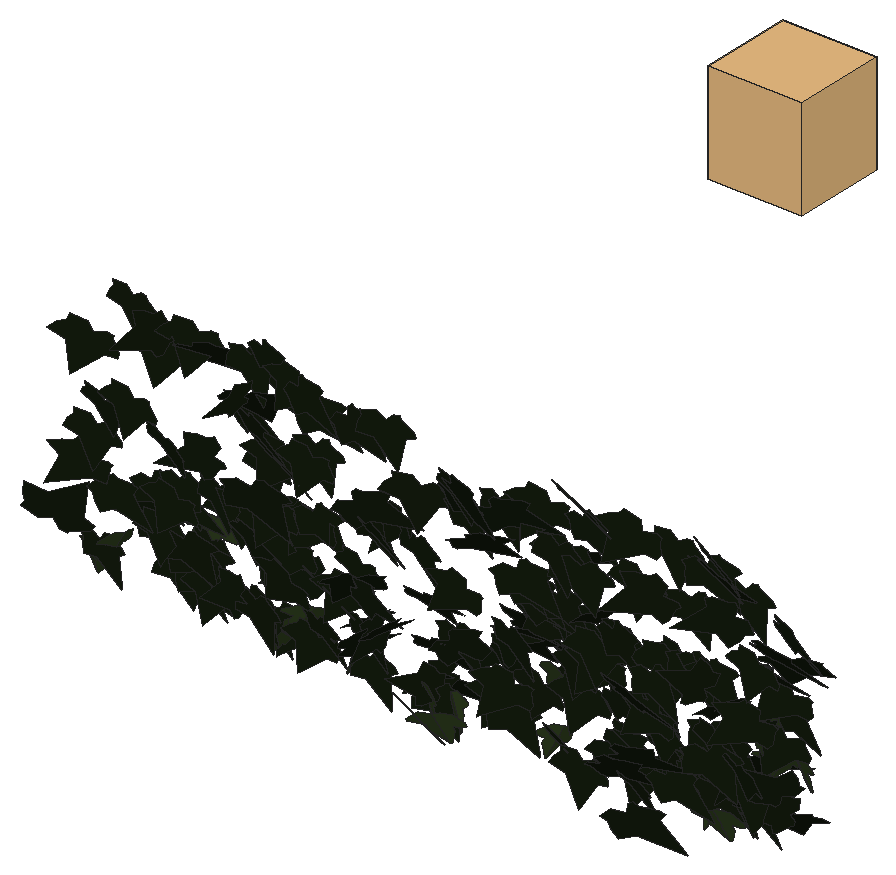
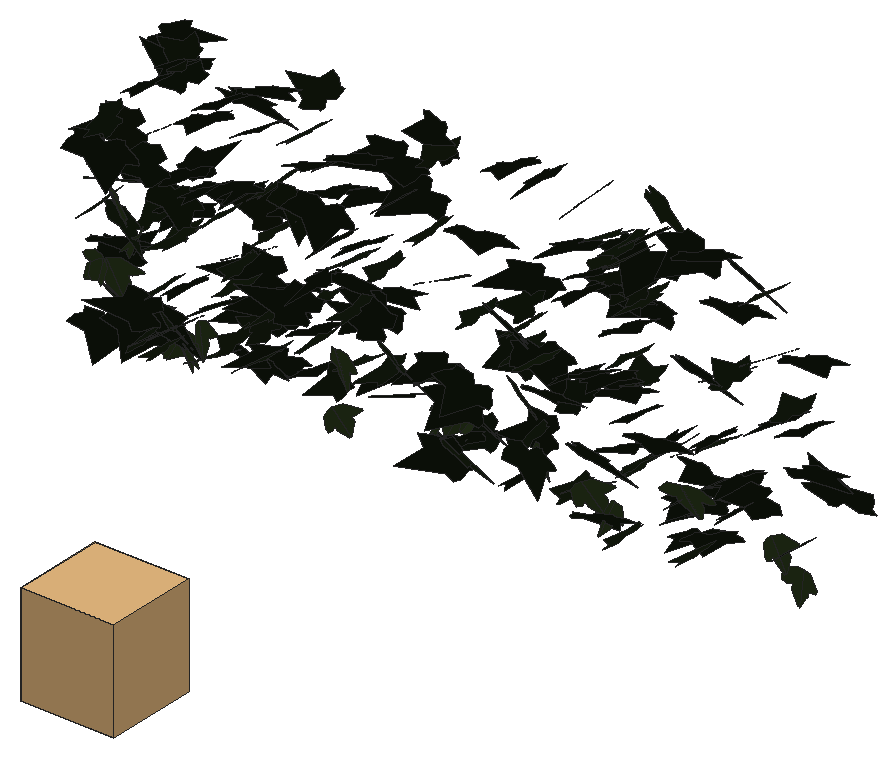
# SketchUp Ruby script. Lengths in millimetres.
U = 1.mm
M = Sketchup.active_model
def pt(a) = Geom::Point3d.new(a.map { |v| v * U })
def face(e, loops, mat)
  f = e.add_face(loops[0].map { |a| pt(a) })
  loops[1..].each { |l| e.add_face(l.map { |a| pt(a) }).erase! }
  f.material = f.back_material = mat if mat
  f
end
# faces: each face lists its corners as indices into pts; further lists are holes
def faces(e, pts, list, mat = nil) = list.each { |f| face(e, (f[0].is_a?(Array) ? f : [f]).map { |l| l.map { |i| pts[i] } }, mat) }
# xy, xz, yz: faces in a plane at the given z, y or x. An outline is a flat list of corners, or four numbers for a rectangle; further outlines are holes
def ring(l) = l.size == 4 ? [[l[0], l[1]], [l[2], l[1]], [l[2], l[3]], [l[0], l[3]]] : l.each_slice(2).to_a
def flat(e, list, mat, &to3) = list.each { |f| face(e, (f[0].is_a?(Array) ? f : [f]).map { |l| ring(l).map { |u, v| to3.(u, v) } }, mat) }
def xy(e, z, list, mat = nil) = flat(e, list, mat) { |x, y| [x, y, z] }
def xz(e, y, list, mat = nil) = flat(e, list, mat) { |x, z| [x, y, z] }
def yz(e, x, list, mat = nil) = flat(e, list, mat) { |y, z| [x, y, z] }
def lines(e, pts, list) = list.each { |a, b| e.add_line(pt(pts[a]), pt(pts[b])) }
# prism: a flat outline (further loops are holes) pulled along v
def prism(e, loops, v, mat = nil)
  f = face(e, loops, mat); d = Geom::Vector3d.new(v.map { |x| x * U })
  f.pushpull(f.normal.samedirection?(d) ? d.length : -d.length)
end
def box(e, o, s, mat = nil) = prism(e, [[o, [o[0] + s[0], o[1], o[2]], [o[0] + s[0], o[1] + s[1], o[2]], [o[0], o[1] + s[1], o[2]]]], [0, 0, s[2]], mat)
def at(x, y, z, deg = 0) = Geom::Transformation.translation(pt([x, y, z])) * Geom::Transformation.rotation(ORIGIN, Z_AXIS, deg.degrees)
def axes(o, x, y, z) = Geom::Transformation.new([*x, 0, *y, 0, *z, 0, *pt(o).to_a, 1])
def part(name) = M.definitions.add(name)
# library, detail: a bought-in or finely detailed component or shape, given as its bounding box
def library(name, o, s) = part(name).tap { |d| box(d.entities, o, s) }
def detail(e, o, s) = box(e.add_group.entities, o, s)
def put(e, d, t, mat = nil) = e.add_instance(d, t).tap { |i| i.material = mat if mat }
def group(e, t, mat = nil) = e.add_group.tap { |g| g.transformation = t; g.material = mat if mat }.entities
root = M.entities
M.materials.add("efeu1").color = [18, 25, 13]
M.materials.add("efeu2").color = [43, 57, 29]
c1 = part("ivyleaf_9")
p = [[39.1,54.8,31.7],[34.5,51.8,30.2],[-5.3,25.2,17.3],[-17.9,28.3,20.9],[-21.6,21.7,17],[-20.2,4.3,5.3],
  [-22.9,-0.3,2.5],[-17.1,-4,-0.6],[-2,-2.1,-1.2],[-0.7,-15.4,-10.1],[16.6,-22.3,-16.7],[21.1,-15.1,-12.5],
  [32.7,-10.7,-11],[46.1,-1.8,-6.6],[30.8,11.2,3.8]]
faces(c1.entities,p,[[0,1,2,3,4,5,6,7,8,9,10,11,12,13,14]],"efeu1")
c2 = part("ivyleaf_10")
p = [[0,12.8,-0.8],[-1.5,51.3,-10.9],[-4.9,51,-11.6],[-13.6,26.5,-7.3],[-13.2,15.9,-4.6],[-21.1,19.3,-7.2],
  [-29.5,16.3,-8.3],[-29.2,8.3,-6.2],[-19.7,-9.8,0.5],[-7.6,-13,4],[1,-12.2,5.8],[-0.4,51.1,-11.1],
  [-1.5,51.1,-10.9],[1,-12.4,5.9],[16.9,-12.4,3.5],[35.1,9.1,-5.1],[35,12.9,-6.1],[20.5,16.4,-4.9],
  [15.8,15,-3.8],[15.3,27.6,-7.1],[12.8,31.3,-7.8]]
faces(c2.entities,p,[[0,1,2,3,4,5,6,7,8,9,10],[11,12,0,13,14,15,16,17,18,19,20]],"efeu2")
c3 = library("Spot Light\#4",[-129.6,-129.6,-280.7],[259.2,259.2,280.7])
put(root,c1,axes([4198.2,621.9,4453],[-2.17521,-0.56393,0.28451],[-0.49117,-0.11993,-1.27446],[1.09721,-1.17168,-0.00648]))
put(root,c2,axes([4187.2,653,4207.9],[-1.96458,0.66362,0.3006],[-0.53689,0.11655,-1.22602],[-1.27837,-1.06879,0.05295]))
put(root,c1,axes([4182.6,644.8,4747.2],[-1.77094,-0.96735,-0.03453],[0.07015,0.01245,-1.34212],[1.8409,-0.93106,0.01792]))
put(root,c1,axes([4173.7,525.1,4344.4],[-1.68412,0.35327,1.1592],[1.86407,-0.63675,0.94171],[1.35815,1.31199,0.14491]))
put(root,c1,axes([4219.9,612.5,4546.3],[-0.69913,-1.27771,0.14771],[-0.04871,-0.14633,-1.32938],[2.44746,-0.3679,0.01574]))
put(root,c1,axes([4222.4,626.1,4254.8],[0.32814,-1.25535,-0.14444],[-0.04891,0.14227,-1.26712],[2.40445,0.17422,-0.00606]))
put(root,c1,axes([4221.1,638.4,4594.8],[-0.17399,-1.04647,0.79155],[0.40634,-0.79476,-1.02606],[2.46395,0.05717,0.22511]))
put(root,c2,axes([4255.4,654.6,4265.7],[-0.51962,-1.21507,0.10633],[-0.08084,-0.09942,-1.24521],[2.31995,-0.27561,-0.01957]))
put(root,c1,axes([4288.6,655.5,4871.3],[-0.21454,-1.27477,0.33346],[0.08333,-0.33811,-1.27777],[2.50639,-0.09788,0.07102]))
put(root,c1,axes([4293.9,651.4,4365.3],[0.7941,0.11418,-1.19805],[1.20217,1.05853,0.32087],[1.9496,-0.69922,0.29012]))
put(root,c1,axes([4324.5,678.6,4416.3],[0.2224,-1.03055,-0.76501],[-0.07622,0.76487,-1.03649],[2.4415,0.11775,0.03733]))
put(root,c1,axes([4341.9,586.1,4664.6],[-0.84168,-1.19771,0.44407],[-0.01634,-0.46713,-1.26846],[2.43106,-0.41781,0.14522]))
put(root,c1,axes([4339.5,666.6,4331.3],[0.44349,-1.20813,-0.37403],[-0.07039,0.37366,-1.22996],[2.40596,0.23363,0.03296]))
put(root,c1,axes([4343,505.4,4484],[0.73383,-1.04531,-0.7256],[0.10638,0.77136,-1.08154],[2.41942,0.28313,0.26763]))
put(root,c1,axes([4421.8,580.6,4863.1],[-2.42111,0.60102,-0.08894],[0.14414,-0.0479,-1.40691],[-1.14729,-1.27433,0.01093]))
put(root,c1,axes([4395.2,634,4803],[-1.87419,-0.84722,-0.36204],[0.67064,0.14329,-1.29379],[1.62017,-1.03937,0.11674]))
put(root,c1,axes([4402.9,619.3,4363.2],[-0.63281,-1.20454,0.19011],[-0.08931,-0.18427,-1.24958],[2.31914,-0.33577,0.00375]))
put(root,c1,axes([4414,678.9,4241.6],[-0.85109,-1.11859,-0.4356],[0.21682,0.4232,-1.2037],[2.27431,-0.45894,-0.04826]))
put(root,c1,axes([4429.1,644.8,4468.3],[0.16814,-1.26485,-0.32961],[-0.13151,0.32538,-1.26714],[2.48418,0.10283,-0.04477]))
put(root,c1,axes([4422.5,595.2,4590.1],[0.21836,-1.05693,0.82305],[0.54807,-0.78729,-1.05115],[2.48991,0.26599,0.1592]))
put(root,c1,axes([4428.6,707.5,4207.5],[0.7171,-1.19637,-0.10522],[0.02586,0.11451,-1.25341],[2.28557,0.37406,0.04719]))
put(root,c2,axes([4463.7,707.8,4347.6],[2.32206,0.04788,-0.28919],[-0.5535,0.04286,-1.21988],[-0.06979,1.25315,0.05277]))
put(root,c1,axes([4429.4,619.1,4443.4],[1.28685,-0.93162,-0.66201],[0.11275,0.79673,-1.0607],[2.17221,0.51055,0.44724]))
put(root,c1,axes([4447.2,678.8,4236.6],[0.09817,-1.01345,-0.78375],[0.23939,0.7846,-1.00627],[2.4265,-0.0364,0.13098]))
put(root,c1,axes([4468,653.2,4298.1],[-0.5128,-0.92664,-0.92044],[0.77281,0.83381,-0.9583],[2.36256,-0.47387,0.11368]))
put(root,c1,axes([4481.1,687.8,4315.1],[-0.22243,-1.20869,0.31111],[-0.13571,-0.3055,-1.21366],[2.37149,-0.13085,-0.04027]))
put(root,c1,axes([4465.7,612.9,4346],[-0.80442,-0.47061,-1.11979],[2.02948,0.42397,-0.58068],[1.10696,-1.1193,0.25087]))
put(root,c1,axes([4547.4,601.6,4588.6],[-2.29914,0.44614,0.26944],[-0.49616,0.0717,-1.28759],[-0.85892,-1.23564,0.02257]))
put(root,c1,axes([4506,606,4876.9],[-1.42236,-1.12046,-0.07532],[0.06806,0.06669,-1.34682],[2.13619,-0.74817,-0.00724]))
put(root,c1,axes([4491.3,701,4446.1],[0.0135,-1.25666,0.16762],[-0.06924,-0.16776,-1.25614],[2.41187,0.00222,-0.037]))
put(root,c1,axes([4521.3,646.8,4236.8],[-0.82066,-1.17383,0.45924],[-0.17031,-0.45564,-1.24864],[2.39287,-0.43501,0.06863]))
put(root,c1,axes([4530.3,502.8,4518.2],[-1.11825,-1.04687,0.60097],[-0.11015,-0.64318,-1.17699],[2.29472,-0.54103,0.23637]))
put(root,c1,axes([4525.5,574.4,4862.4],[2.25203,0.61737,0.26006],[0.44223,0.11684,-1.33465],[-1.19581,1.20588,-0.00382]))
put(root,c1,axes([4559.2,694.6,4435.6],[-1.56947,-0.82912,-0.47806],[0.9349,0.17492,-1.15071],[1.56327,-0.93701,0.20821]))
put(root,c1,axes([4621.2,609.4,4738.4],[1.52482,-0.87049,-0.63857],[-0.3957,0.65591,-1.15498],[2.01622,0.78706,0.25626]))
put(root,c1,axes([4627.6,711.6,4180],[0.47682,-1.21851,0.13044],[0.03168,-0.12975,-1.24396],[2.33211,0.2509,-0.00977]))
put(root,c1,axes([4666.8,546.1,4310.7],[-0.71611,-0.3566,1.25662],[-1.27586,-1.06965,-0.50427],[2.13367,-0.75929,0.12022]))
put(root,c1,axes([4652,643.4,4446.1],[-0.25147,-1.30218,0.02339],[-0.01076,-0.02293,-1.30886],[2.47869,-0.13221,-0.00331]))
put(root,c1,axes([4671,686.7,4374.2],[-1.28492,-1.0514,0.26656],[-0.07988,-0.28842,-1.24393],[2.06278,-0.66609,0.11787]))
put(root,c1,axes([4653,607.9,4869.3],[-0.0984,-1.35294,-0.0195],[0.00207,0.01948,-1.35393],[2.57519,-0.05171,0.00034]))
put(root,c1,axes([4647.6,655.3,4846.4],[0.62704,-1.24322,-0.31249],[0.01769,0.32496,-1.28301],[2.43964,0.31718,0.08962]))
put(root,c1,axes([4657.1,660.4,4587.8],[-0.14463,-1.23712,0.38307],[0.10814,-0.38655,-1.23707],[2.46241,-0.05569,0.07683]))
put(root,c1,axes([4680.9,666.1,4503.6],[-1.39953,-1.04333,0.06805],[-0.0321,-0.07135,-1.27614],[1.98962,-0.73504,0.02728]))
put(root,c3,at(4681.1,2446,4806.3))
put(root,c1,axes([4655.1,649.7,4871.7],[1.0809,-1.17667,-0.19996],[-0.08032,0.20151,-1.30565],[2.27013,0.56739,0.04901]))
put(root,c1,axes([4679.1,565.6,4799.8],[2.15943,0.88787,-0.20203],[-0.31028,-0.11948,-1.44072],[-1.70499,1.14627,0.00631]))
put(root,c1,axes([4665.2,591.3,4295.3],[0.72383,-1.35861,-0.05097],[-0.0282,0.04878,-1.41084],[2.58737,0.38061,-0.00112]))
put(root,c1,axes([4668.8,587.6,4727],[1.22943,-1.18876,0.24908],[0.19959,-0.22647,-1.35284],[2.30294,0.65425,-0.01572]))
put(root,c1,axes([4686.5,583,4284.4],[0.30938,-1.39094,0.187],[-0.01497,-0.18915,-1.40009],[2.671,0.16005,-0.02951]))
put(root,c1,axes([4720.8,702.8,4194.2],[-1.8468,-0.78716,0.04801],[0.12187,-0.15452,-1.23918],[1.49596,-0.95919,0.16022]))
put(root,c2,axes([4710.2,647.7,4188.9],[-0.14665,-0.87526,-0.91098],[0.53193,0.87825,-0.86745],[2.34477,-0.25398,0.13981]))
put(root,c1,axes([4745.7,460.8,4867.2],[-1.6426,1.00778,-0.3785],[0.42183,-0.30838,-1.32648],[-2.00493,-0.89054,0.03101]))
put(root,c1,axes([4770.7,684.2,4332.9],[-2.24847,0.30894,0.32486],[-0.59642,0.08569,-1.22114],[-0.61014,-1.22227,-0.0035]))
put(root,c1,axes([4717.6,551.2,4461.4],[-0.73834,-0.87853,0.97421],[0.43475,-1.04564,-0.85198],[2.45853,-0.07893,0.44323]))
put(root,c2,axes([4755.3,683.8,4239.7],[-0.97077,-1.02092,0.52289],[-0.27127,-0.51141,-1.13754],[2.16612,-0.52158,0.09188]))
put(root,c1,axes([4772.8,575.9,4684.8],[-2.29057,-0.51015,-0.24264],[0.4059,0.11847,-1.30694],[0.99558,-1.22202,-0.02541]))
put(root,c1,axes([4743.1,613.9,4495.7],[-0.11946,-1.19796,-0.55241],[0.20864,0.54639,-1.19735],[2.502,-0.10276,0.07347]))
put(root,c1,axes([4768.1,633,4834.1],[-1.31021,-0.9011,0.6956],[-0.16576,-0.76883,-1.08217],[2.16016,-0.60555,0.33886]))
put(root,c1,axes([4776.1,538,4569.9],[-1.11249,-1.1918,0.42443],[-0.31188,-0.39228,-1.32721],[2.3875,-0.60658,0.0244]))
put(root,c1,axes([4735.3,558.3,4695.8],[1.44969,-1.13179,0.51572],[0.53232,-0.43338,-1.36421],[2.30648,0.81139,-0.00929]))
put(root,c1,axes([4788.9,576,4457.8],[-1.89015,-0.87565,-0.0172],[0.02347,0.01202,-1.32404],[1.66669,-0.99322,-0.00086]))
put(root,c1,axes([4749.4,491.3,4627.1],[-1.08951,-0.39235,-1.2628],[1.95688,0.7332,-0.69392],[1.58251,-1.17677,-0.01132]))
put(root,c1,axes([4797.7,647.4,4494.5],[-1.39903,-0.97402,0.41867],[-0.2092,-0.4367,-1.20895],[2.00687,-0.72453,0.16584]))
put(root,c1,axes([4803.3,648.9,4207.7],[-1.08796,-1.06868,0.43413],[-0.23206,-0.42582,-1.20878],[2.18304,-0.57786,0.08786]))
put(root,c1,axes([4784.6,679.9,4226.2],[0.78188,-1.15155,0.26388],[0.18512,-0.24546,-1.22261],[2.24081,0.42209,0.00893]))
put(root,c1,axes([4791.8,654.5,4509.4],[0.42885,-1.16194,-0.53232],[0.15788,0.55268,-1.17128],[2.4273,0.16934,0.17023]))
put(root,c1,axes([4812.1,635.7,4690.8],[-0.11072,-1.31597,-0.24903],[-0.03056,0.24993,-1.31699],[2.54882,-0.05417,-0.02661]))
put(root,c1,axes([4843.3,577.1,4698.3],[-0.99812,-1.14335,0.3608],[-0.11115,-0.36897,-1.25416],[2.27909,-0.51872,0.09684]))
put(root,c1,axes([4822.1,617,4798.9],[0.51809,-0.95711,-0.88866],[0.41506,0.92832,-0.93302],[2.45078,0.04511,0.34588]))
put(root,c1,axes([4840.9,544.5,4884.4],[1.02518,-1.10963,-0.68],[-0.44576,0.64127,-1.23197],[2.43641,0.58423,0.06073]))
put(root,c1,axes([4848.3,593.7,4387.5],[0.72853,-0.93172,0.93945],[0.90495,-0.81577,-1.00281],[2.34995,0.603,0.09492]))
put(root,c1,axes([4911.7,688,4277.2],[0.28555,1.27275,-0.06793],[-0.01066,-0.06774,-1.28156],[-2.42572,0.15012,-0.00236]))
put(root,c1,axes([4929.5,615.3,4389.5],[-2.17985,-0.51639,-0.17128],[0.48712,-0.15916,-1.23167],[0.91371,-1.14711,0.248]))
put(root,c2,axes([4932.6,629.1,4237],[0.82258,-1.13409,0.29773],[0.20642,-0.27729,-1.21366],[2.22197,0.4456,0.00252]))
put(root,c1,axes([4978.6,563.5,4452.7],[0.57934,1.14447,-0.73418],[-0.36633,-0.7085,-1.18425],[-2.56174,0.36014,0.00332]))
put(root,c1,axes([4935.9,648,4284.3],[0.61149,-1.2243,0.35256],[0.15775,-0.34274,-1.26574],[2.41963,0.33175,-0.00658]))
put(root,c1,axes([4945.8,656.7,4198.8],[0.20015,-1.30888,-0.29519],[-0.08566,0.29249,-1.31293],[2.5522,0.11246,-0.02092]))
put(root,c1,axes([4951.6,618.2,4453.6],[-0.41986,-1.11031,0.60959],[0.16828,-0.63076,-1.11686],[2.4048,-0.14971,0.18459]))
put(root,c1,axes([4944.9,580.2,4263],[0.79218,0.36053,1.25445],[1.74761,0.85487,-0.55037],[-1.76542,1.00802,0.01808]))
put(root,c1,axes([4949.8,640.8,4564.1],[0.7669,-1.21226,-0.24904],[-0.09611,0.24558,-1.27715],[2.35339,0.40507,0.029]))
put(root,c1,axes([4991.2,318.3,4555.7],[-1.38603,-0.69552,1.1133],[-0.06726,-1.2623,-0.81172],[2.49743,-0.42,0.596]))
put(root,c1,axes([5014.4,667.3,4569.5],[-2.17905,0.21205,-0.56374],[1.00198,-0.23585,-1.15795],[-0.55682,-1.25422,0.12243]))
put(root,c1,axes([4990.5,524.5,4873.4],[0.78902,-0.9867,-0.84246],[-0.3899,0.82354,-1.06536],[2.43829,0.45099,0.10225]))
put(root,c1,axes([4976,599.6,4580.5],[1.35017,-1.03812,0.32015],[0.32257,-0.27192,-1.2573],[2.04226,0.72927,-0.01307]))
put(root,c1,axes([4976.2,569.3,4640.5],[0.39665,-0.07674,-1.38118],[0.83252,1.32875,-0.00782],[2.49762,-0.43072,0.22195]))
put(root,c1,axes([5035.6,575.1,4339.2],[-1.94864,0.55738,-0.66076],[1.07879,-0.34044,-1.16551],[-1.24216,-1.17005,0.02435]))
put(root,c1,axes([5010.8,536.6,4446.7],[1.69584,-0.72957,-0.67448],[-0.58515,0.65904,-1.11906],[1.79816,0.90252,0.27194]))
put(root,c1,axes([5069.9,552.6,4880.6],[-0.44423,-1.27695,-0.30092],[0.10736,0.2956,-1.2981],[2.49455,-0.24012,0.00228]))
put(root,c1,axes([5069.8,686,4389.1],[2.33781,0.21743,-0.26564],[-0.52851,0.04919,-1.24385],[-0.38406,1.25579,0.09472]))
put(root,c1,axes([5076.1,501.1,4379.1],[1.08034,0.58795,1.0697],[1.07251,0.92024,-0.80484],[-2.06073,0.78717,0.14191]))
put(root,c1,axes([5078.4,652.6,4543],[0.37237,-1.25727,0.37387],[0.17066,-0.3643,-1.27201],[2.49054,0.21294,0.03127]))
put(root,c1,axes([5136.7,687.3,4218.7],[-2.02226,0.63676,-0.30987],[0.29098,-0.33928,-1.22149],[-1.31598,-1.05353,0.20608]))
put(root,c1,axes([5122.7,605.6,4712.3],[-1.69836,-0.80246,-0.52832],[0.7927,0.32666,-1.19967],[1.64777,-0.98425,0.03258]))
put(root,c1,axes([5180.5,577.7,4246.4],[-1.53447,0.80915,0.54487],[-0.71444,0.3951,-1.14221],[-1.71361,-0.88929,-0.0117]))
put(root,c1,axes([5125.3,647.5,4309.9],[2.31188,0.3756,-0.03514],[-0.06365,-0.01078,-1.27148],[-0.71513,1.21519,-0.00042]))
put(root,c1,axes([5123.9,551.2,4197.3],[2.08378,-0.57027,-0.27413],[-0.43558,0.15384,-1.23413],[1.12268,1.11815,0.02998]))
put(root,c1,axes([5117,689.3,4193.6],[2.21814,0.13479,0.4986],[0.93696,0.08229,-1.17302],[-0.2973,1.26498,0.02318]))
put(root,c2,axes([5159,584.2,4229.1],[-0.96697,1.01692,-0.54611],[0.34395,-0.51923,-1.13501],[-2.16974,-0.53551,0.06346]))
put(root,c1,axes([5152.6,627.8,4204.3],[-0.18253,-1.18698,-0.55787],[0.06122,0.55706,-1.19079],[2.49538,-0.10049,-0.01159]))
put(root,c1,axes([5187.2,652.5,4359],[0.41302,-1.24933,-0.14827],[0.1255,0.16155,-1.2647],[2.39113,0.20732,0.09199]))
put(root,c2,axes([5224.1,534.5,4206.1],[-2.1198,-0.5065,-0.34144],[0.57278,0.16288,-1.22335],[1.01165,-1.15353,-0.02281]))
put(root,c2,axes([5220.8,605.6,4217.6],[-0.3192,1.21082,-0.34158],[0.07086,-0.33967,-1.22234],[-2.39332,-0.17155,0.00937]))
put(root,c1,axes([5208,609.8,4359.4],[0.2025,-0.07283,-1.33171],[0.04762,1.33581,-0.07105],[2.53784,-0.01925,0.10759]))
put(root,c1,axes([5224.8,622.2,4692.6],[0.90889,-1.25207,-0.18062],[-0.10173,0.17292,-1.34],[2.40546,0.4804,0.01158]))
put(root,c1,axes([5270.3,572.9,4525.4],[-1.57561,-0.73034,0.72215],[-0.39876,-0.78794,-1.03707],[1.91363,-0.76552,0.37848]))
put(root,c1,axes([5335.1,657.5,4370.5],[-2.00904,0.65223,-0.3732],[0.55281,-0.23936,-1.23989],[-1.319,-1.09375,0.04879]))
put(root,c1,axes([5294,525.9,4802.4],[-0.10903,-1.07996,0.85608],[0.48775,-0.85023,-1.05542],[2.57708,0.11523,0.23597]))
put(root,c1,axes([5328.9,641.7,4252.4],[-1.50218,-0.92994,0.32794],[0.05774,-0.44276,-1.18252],[1.87581,-0.73109,0.29902]))
put(root,c1,axes([5299.2,671.9,4342.7],[1.50986,-1.01362,-0.28741],[-0.14541,0.30348,-1.2812],[1.9999,0.78732,0.12383]))
put(root,c1,axes([5322.9,635,4735.9],[0.23008,-1.33246,-0.04934],[-0.03737,0.04776,-1.33785],[2.53741,0.12152,-0.01523]))
put(root,c1,axes([5311.9,484.4,4832.3],[-0.02648,0.03691,-1.4553],[2.77057,0.0082,-0.01371],[0.01494,-1.45534,-0.03698]))
put(root,c1,axes([5335.1,510,4698.8],[2.12394,0.7508,0.52686],[0.83504,0.29168,-1.34504],[-1.53297,1.19913,-0.0027]))
put(root,c1,axes([5342.3,667.8,4429.4],[1.19644,-0.57449,0.99092],[1.39674,-0.66583,-0.8516],[1.67369,0.96633,0.00232]))
put(root,c1,axes([5380.3,607.3,4441.5],[2.48039,0.37645,0.03702],[0.06761,0.0104,-1.35655],[-0.71673,1.30376,0.00013]))
put(root,c1,axes([5383.3,590.7,4258.8],[-0.00447,-1.10531,-0.68086],[0.23731,0.67752,-1.10032],[2.45927,-0.06739,0.10494]))
put(root,c1,axes([5392.7,676.1,4460.9],[1.08954,-1.16183,-0.0931],[-0.0884,0.08091,-1.2952],[2.21653,0.57433,-0.00589]))
put(root,c1,axes([5384,537,4781.3],[0.13141,0.21885,-1.43136],[1.04973,1.32098,0.22858],[2.54806,-0.55549,-0.02035]))
put(root,c1,axes([5419.2,657.7,4303.2],[-0.80671,-1.07127,0.62758],[0.01297,-0.66514,-1.13079],[2.36291,-0.36209,0.22047]))
put(root,c2,axes([5442.8,679.6,4323.1],[1.59666,-0.77947,-0.52171],[-0.30155,0.57212,-1.10957],[1.75945,0.8054,0.28327]))
put(root,c2,axes([5445.2,686.2,4184.2],[-0.72322,-1.07178,0.54613],[0.095,-0.58629,-1.11586],[2.28739,-0.31452,0.21902]))
put(root,c1,axes([5423.8,601.1,4584.4],[0.52857,-1.12082,-0.60678],[0.17231,0.6368,-1.13483],[2.41955,0.1995,0.21337]))
put(root,c1,axes([5422.8,540.9,4486.6],[0.61918,-1.26749,0.32696],[0.15657,-0.31645,-1.30857],[2.48632,0.33557,0.00098]))
put(root,c1,axes([5476.5,641.5,4495.6],[-2.39039,-0.35142,0.02931],[-0.04722,-0.02008,-1.30416],[0.66948,-1.25617,0.01265]))
put(root,c1,axes([5469.2,491.8,4394.6],[-1.81564,-0.84654,0.23753],[-0.37912,-0.13328,-1.27503],[1.62985,-0.97404,-0.03197]))
put(root,c1,axes([5466.1,620.2,4787.8],[-1.72896,-0.9713,0.2073],[-0.10735,-0.23003,-1.32498],[1.88716,-0.90296,0.11455]))
put(root,c1,axes([5434.1,607.5,4546.7],[1.35452,-0.8815,-0.68058],[-0.09566,0.78144,-1.0647],[2.11735,0.59922,0.38728]))
put(root,c1,axes([5460,524.4,4658.7],[0.10465,-0.99872,-0.93345],[0.54873,0.92166,-0.96912],[2.5432,-0.15776,0.24751]))
put(root,c1,axes([5508.7,653,4660],[1.52284,1.02322,-0.25314],[-0.33885,-0.18204,-1.29863],[-1.97727,0.81925,0.02759]))
put(root,c1,axes([5481.7,613.7,4224.8],[1.92255,-0.77261,-0.12133],[-0.17612,0.07872,-1.27174],[1.478,1.01438,0.00628]))
put(root,c1,axes([5499.3,656.3,4499],[0.82296,-0.61036,-1.13884],[-0.66435,1.10108,-0.72267],[2.36767,0.52111,0.19306]))
put(root,c1,axes([5517.2,627.3,4689.8],[-1.09346,-1.19737,0.16548],[-0.03701,-0.17404,-1.32684],[2.3002,-0.572,0.05732]))
put(root,c1,axes([5512.4,687,4333.5],[-0.44076,-1.06441,0.75246],[-0.17497,-0.749,-1.08781],[2.47468,-0.24254,0.0571]))
put(root,c1,axes([5501,612.6,4571.3],[0.63576,-1.10321,-0.59625],[-0.19498,0.59097,-1.15084],[2.37868,0.3433,0.06503]))
put(root,c1,axes([5539.3,633.4,4401],[-0.40739,-1.01009,0.80251],[-0.10368,-0.80568,-1.02861],[2.45309,-0.2018,0.0898]))
put(root,c1,axes([5553.2,641.4,4338.5],[-1.12916,-1.21783,0.29633],[-0.17014,-0.28591,-1.35396],[2.37934,-0.59839,0.04381]))
put(root,c1,axes([5540.8,563.9,4728],[-0.15956,-1.38207,0.15317],[-0.01236,-0.15306,-1.38461],[2.64643,-0.08404,0.00277]))
put(root,c1,axes([5547.2,679.4,4401.8],[0.70023,-0.11223,1.30728],[2.45593,0.27669,-0.33942],[-0.45198,1.32959,0.18098]))
put(root,c1,axes([5602.9,647,4426.7],[-1.55866,-0.913,0.44209],[-0.26077,-0.46342,-1.21086],[1.91291,-0.80709,0.19515]))
put(root,c1,axes([5590.7,583.2,4202.3],[-0.64786,-1.32051,0.19637],[-0.10454,-0.18863,-1.36367],[2.53869,-0.34475,-0.00604]))
put(root,c1,axes([5587.8,595.9,4798.5],[0.77309,-1.22151,-0.33495],[0.02926,0.35648,-1.28139],[2.41041,0.38745,0.12298]))
put(root,c1,axes([5602,563.7,4698.5],[-0.68415,-1.24355,-0.26908],[0.62085,0.18018,-1.26853],[2.34055,-0.41129,0.25784]))
put(root,c1,axes([5583.4,556.9,4865.8],[0.68678,-0.99137,0.89218],[0.98827,-0.7469,-1.03996],[2.33804,0.60692,0.17751]))
put(root,c1,axes([5640.5,568.6,4597.3],[0.70644,1.26574,0.06994],[0.04834,0.06543,-1.31903],[-2.41215,0.372,-0.00595]))
put(root,c1,axes([5633.4,635.8,4366.1],[1.41068,-0.91425,-0.59007],[-0.47229,0.55312,-1.16873],[2.01637,0.76918,0.13907]))
put(root,c1,axes([5635,651.1,4261.3],[1.39552,-0.84139,-0.73851],[-0.33566,0.78497,-1.06944],[2.10407,0.68328,0.31921]))
put(root,c1,axes([5631.2,636.9,4241.6],[0.4056,-0.46274,-1.28453],[0.85987,1.25074,-0.37561],[2.45211,-0.36205,0.34418]))
put(root,c1,axes([5674.7,541.5,4547.3],[-1.15592,-1.15631,-0.13362],[0.12895,0.11534,-1.3061],[2.21158,-0.61109,0.00632]))
put(root,c1,axes([5662.6,626.5,4532.5],[0.28917,-1.31759,0.25893],[0.07528,-0.25607,-1.32629],[2.55449,0.1567,0.00978]))
put(root,c1,axes([5718.7,636.9,4212],[-2.08416,-0.1847,-0.62254],[1.15704,0.13734,-1.11015],[0.43433,-1.25216,-0.02993]))
put(root,c1,axes([5752.8,578.6,4834.7],[-1.90703,-0.86953,0.39492],[-0.39061,-0.36297,-1.31993],[1.77511,-1.01402,0.13382]))
put(root,c1,axes([5722.9,530.2,4596.3],[1.02527,-1.31162,-0.38333],[-0.24464,0.36157,-1.41783],[2.58917,0.55355,0.01783]))
put(root,c1,axes([5725.2,687.9,4261.7],[0.4412,-1.144,0.52617],[0.16822,-0.51891,-1.16716],[2.39061,0.24765,-0.01498]))
put(root,c1,axes([5718.3,500.3,4280.1],[2.25026,0.20201,0.70448],[1.32151,0.11895,-1.19949],[-0.44616,1.37117,0.00027]))
put(root,c1,axes([5734.2,559.3,4235.3],[0.85988,-1.18045,0.63929],[0.52632,-0.57821,-1.26312],[2.50014,0.52772,0.04604]))
put(root,c1,axes([5764.4,571.6,4729.3],[-0.70054,-1.28406,0.32494],[-0.04119,-0.33138,-1.33402],[2.52052,-0.3623,0.06851]))
put(root,c1,axes([5749,632.6,4420.6],[0.74701,-1.23269,0.17099],[0.08037,-0.166,-1.29363],[2.36716,0.39464,-0.01004]))
put(root,c1,axes([5803.4,575.5,4403.8],[-1.45221,-0.75243,0.82337],[-0.5608,-0.82617,-1.02807],[2.04738,-0.76,0.30241]))
put(root,c1,axes([5789.4,706.3,4210.3],[-0.92016,-1.06031,0.46299],[0.09244,-0.51994,-1.14002],[2.20002,-0.42163,0.24154]))
put(root,c1,axes([5784.9,615.1,4343.8],[-0.38608,-1.13699,0.59075],[0.17626,-0.60956,-1.14138],[2.4322,-0.13631,0.17649]))
put(root,c2,axes([5806.5,703.3,4275.5],[-0.00615,-1.20526,-0.37549],[0.10058,0.37503,-1.20425],[2.40049,-0.0188,0.0495]))
put(root,c1,axes([5765.2,493.1,4483.2],[1.41917,-0.8168,0.88263],[1.30023,-0.56696,-1.10184],[1.88356,1.00679,0.09558]))
put(root,c1,axes([5814.4,644.8,4519.8],[-0.35753,-1.15985,0.59786],[-0.14041,-0.59361,-1.1748],[2.47945,-0.20086,0.01968]))
put(root,c1,axes([5815.9,630.6,4806.7],[-0.55943,-1.31968,0.07818],[0.00058,-0.08016,-1.3519],[2.51601,-0.29341,0.0177]))
put(root,c1,axes([5777.9,493,4327.5],[1.92282,0.04668,0.96525],[1.82655,0.11508,-1.0101],[-0.2154,1.39255,0.05112]))
put(root,c1,axes([5870.1,503,4749.9],[-2.59938,-0.0259,0.33043],[-0.62875,-0.00669,-1.36604],[0.0509,-1.40518,0.00041]))
put(root,c1,axes([5832.5,520.9,4534.1],[0.21257,-1.19892,-0.53814],[-0.0873,0.53619,-1.20411],[2.49958,0.12068,0.00371]))
put(root,c1,axes([5818.1,460.6,4207.6],[-0.01193,-0.34959,-1.30411],[1.35913,1.10591,-0.29989],[2.18074,-0.69116,0.17977]))
put(root,c1,axes([5848.6,572.7,4560.6],[-1.32008,-1.22984,-0.3321],[0.31451,0.28807,-1.41194],[2.40397,-0.71302,0.00236]))
put(root,c1,axes([5847.4,560.4,4267.8],[0.8395,-1.0599,-0.73058],[0.16415,0.79488,-1.10111],[2.44449,0.31062,0.32484]))
put(root,c1,axes([5875.5,667.2,4347.9],[0.12194,-1.26811,-0.30251],[-0.09526,0.30026,-1.26928],[2.47936,0.0739,-0.03389]))
put(root,c2,axes([5893.3,655.2,4179.2],[1.51392,-0.92167,0.22736],[0.27072,-0.17755,-1.21744],[1.7863,0.80804,-0.00818]))
put(root,c1,axes([5878.4,594.2,4552.5],[0.13549,-1.25881,-0.39591],[0.08417,0.39854,-1.25921],[2.51005,0.05458,0.06359]))
put(root,c1,axes([5897.3,576.7,4716.9],[-0.35628,-1.23719,-0.45577],[0.16113,0.44811,-1.25118],[2.50414,-0.20485,0.01566]))
put(root,c1,axes([5946.2,643.6,4237.2],[-1.29244,1.04755,-0.01213],[0.01108,-0.01068,-1.24841],[-1.99379,-0.67911,0.00092]))
put(root,c1,axes([5890.5,659,4455.9],[1.26181,-1.04852,-0.38198],[0.01876,0.44979,-1.21756],[2.12376,0.619,0.2377]))
put(root,c1,axes([5901.6,644.7,4230.5],[1.01735,-1.03447,-0.68023],[-0.09376,0.72256,-1.13756],[2.35444,0.47576,0.24863]))
put(root,c1,axes([5904.5,696.3,4196.5],[0.82075,-1.19203,-0.13145],[-0.02881,0.13427,-1.26726],[2.28224,0.43038,0.03128]))
put(root,c2,axes([5930.7,619.9,4179.3],[-2.31723,0.04484,-0.25395],[0.48349,-0.00225,-1.21835],[-0.08442,-1.24374,-0.00695]))
put(root,c1,axes([5974.8,663.1,4244.5],[0.4961,0.23996,-1.31938],[-2.10668,-0.72024,-0.34969],[-1.44076,1.13576,0.057]))
put(root,c1,axes([5963.3,532.6,4542.5],[-0.09477,0.04257,1.41718],[-2.06955,-0.9111,-0.01084],[1.73154,-1.08663,0.06461]))
put(root,c1,axes([5923.8,675.4,4332.2],[0.88434,-1.16887,-0.33838],[-0.11891,0.33882,-1.25617],[2.31287,0.46434,0.0648]))
put(root,c1,axes([5947.5,698.4,4206.8],[-0.15516,-1.26472,0.13322],[0.02921,-0.13446,-1.26712],[2.42015,-0.07946,0.02383]))
put(root,c1,axes([5946.1,574.4,4562.3],[0.20724,-1.09654,-0.71782],[0.11062,0.72362,-1.09659],[2.49187,0.05907,0.10838]))
put(root,c1,axes([5989.5,566.6,4492],[0.3758,1.30743,-0.17125],[-0.06266,-0.16821,-1.32224],[-2.50878,0.20005,0.00737]))
put(root,c1,axes([5952.5,567.9,4826.5],[-0.03332,-1.13637,-0.71638],[0.27953,0.71053,-1.13067],[2.5413,-0.09305,0.11498]))
put(root,c1,axes([5950,578.2,4842.3],[0.64778,-0.97262,0.88434],[0.59371,-0.82765,-1.03033],[2.43039,0.46142,0.01599]))
put(root,c1,axes([5967.6,579.8,4397.4],[-0.245,-1.13554,0.68159],[0.10637,-0.68885,-1.13708],[2.51834,-0.08137,0.11434]))
put(root,c1,axes([5946.7,711.4,4270.2],[1.36098,-0.01452,1.03007],[1.8779,0.37006,-0.67978],[-0.56353,1.19811,0.22245]))
put(root,c1,axes([5952.7,579,4791.1],[0.34949,-0.67474,1.26436],[1.52582,-1.00821,-0.65448],[2.26082,0.78474,0.24626]))
put(root,c1,axes([5972.2,692.6,4192.6],[0.94421,-1.15033,0.0306],[0.01963,-0.02888,-1.25275],[2.19,0.49622,-0.00196]))
put(root,c1,axes([6000.4,663.3,4203.1],[1.78887,0.85284,-0.09548],[-0.12209,-0.07138,-1.26914],[-1.6287,0.94207,-0.00973]))
put(root,c1,axes([6014.6,665.8,4242.3],[-1.19283,-1.11366,-0.00561],[0.24722,-0.06671,-1.26955],[2.10507,-0.62321,0.14592]))
put(root,c1,axes([6013.6,491.8,4413.4],[-0.28491,-1.12936,-0.80892],[0.20577,0.80166,-1.13924],[2.63586,-0.18466,0.0015]))
put(root,c2,axes([6027.5,652.6,4403.7],[-0.09859,1.24886,-0.16149],[0.00337,-0.16155,-1.24993],[-2.39662,-0.0516,0.00489]))
put(root,c1,axes([6027.8,605.8,4770.5],[-0.0208,-1.35148,-0.26052],[0.0219,0.26043,-1.3515],[2.6194,-0.01291,0.00923]))
put(root,c1,axes([6002.3,621.7,4580.5],[2.25766,-0.24349,0.56038],[1.08313,-0.005,-1.20689],[0.42313,1.31194,0.09941]))
put(root,c2,axes([6067.4,694.5,4335.8],[-1.64853,-0.87222,0.29976],[-0.43183,-0.19707,-1.22906],[1.70135,-0.89516,-0.0215]))
put(root,c1,axes([6076.9,647.8,4448.4],[-0.63697,1.20466,0.20124],[-0.0604,0.20001,-1.25008],[-2.32369,-0.33542,-0.02267]))
put(root,c1,axes([6093.2,555.9,4493.9],[-2.18595,-0.56951,0.33037],[-0.55874,-0.1516,-1.282],[1.1216,-1.18548,0.00523]))
put(root,c1,axes([6078.1,674.3,4392.3],[-1.79296,-0.86611,-0.0184],[0.20308,-0.08904,-1.27227],[1.63619,-0.93804,0.13776]))
put(root,c1,axes([6074.8,692.6,4189.6],[1.51886,0.9655,-0.09491],[-0.14637,-0.05955,-1.25245],[-1.84058,0.80147,0.02128]))
put(root,c2,axes([6081.5,655.8,4479.3],[1.17099,-1.10104,-0.14151],[-0.11356,0.12876,-1.26125],[2.10968,0.61807,0.01065]))
put(root,c1,axes([6070.1,590.3,4610.4],[-0.75377,-1.12691,0.54071],[-0.13457,-0.5461,-1.18993],[2.37504,-0.38859,0.10419]))
put(root,c1,axes([6119.2,635.1,4236.8],[-1.63954,0.89959,0.31349],[-0.46518,0.19979,-1.24499],[-1.7524,-0.89469,0.03719]))
put(root,c1,axes([6103.8,459.9,4798.2],[-0.21568,-0.52776,-1.3271],[-0.07255,-1.32968,0.53204],[-2.71716,0.07739,0.09113]))
put(root,c1,axes([6120.7,605.4,4300.5],[0.49024,0.15676,1.27165],[-2.21859,-0.50967,0.29895],[1.01207,-1.19319,0.03937]))
put(root,c1,axes([6110.5,655.7,4521.2],[-1.9829,-0.72682,0.36903],[0.04096,-0.62321,-1.16666],[1.55082,-0.91285,0.50266]))
put(root,c1,axes([6079.6,529.1,4375.7],[-0.19716,-0.86687,1.02567],[0.21015,-1.03073,-0.86],[2.54721,0.01794,0.15034]))
put(root,c2,axes([6093.2,700.9,4338],[-1.40793,0.91598,-0.45565],[0.47922,-0.38198,-1.17668],[-1.88718,-0.78036,0.04114]))
put(root,c1,axes([6114.3,656,4607.2],[1.66539,0.89133,-0.58902],[-0.79452,-0.41558,-1.24906],[-1.87167,0.96951,0.00612]))
put(root,c1,axes([6089.1,652.2,4681.9],[1.8627,-0.90264,-0.37513],[-0.51714,0.2587,-1.3314],[1.78704,1.01572,0.00573]))
put(root,c1,axes([6070.8,610.2,4641.7],[2.26471,-0.45056,0.42636],[0.83481,-0.04101,-1.26755],[0.83477,1.26336,0.11091]))
put(root,c1,axes([6102.3,660.4,4479.8],[0.93869,-1.06588,-0.48193],[-0.33097,0.45039,-1.17411],[2.20156,0.52217,0.02897]))
